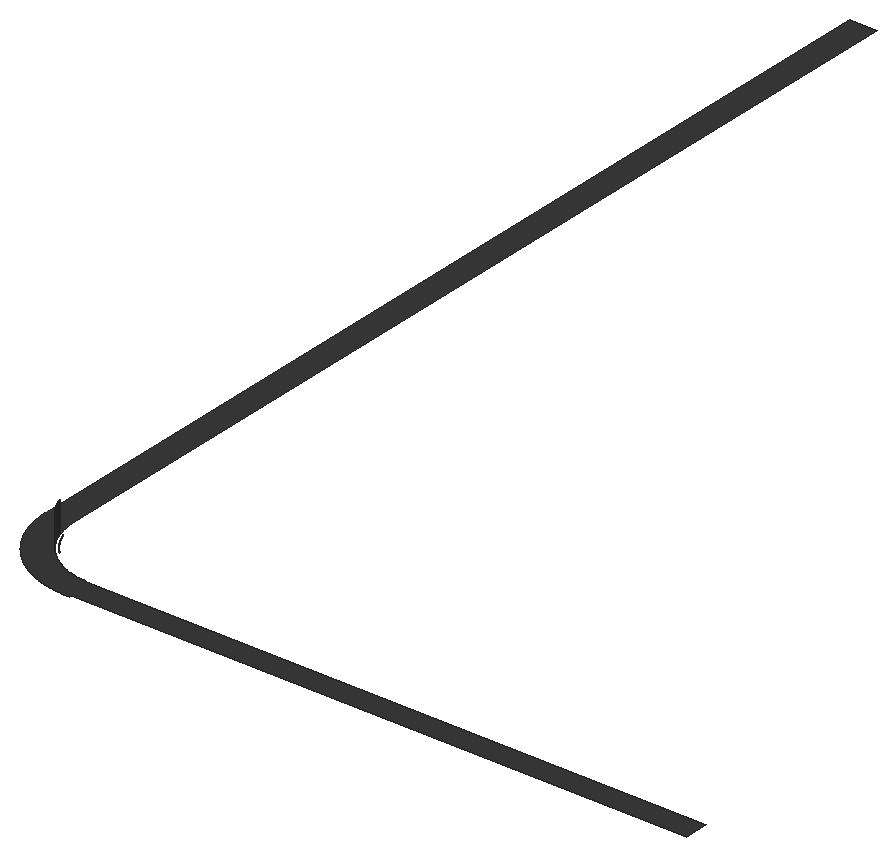
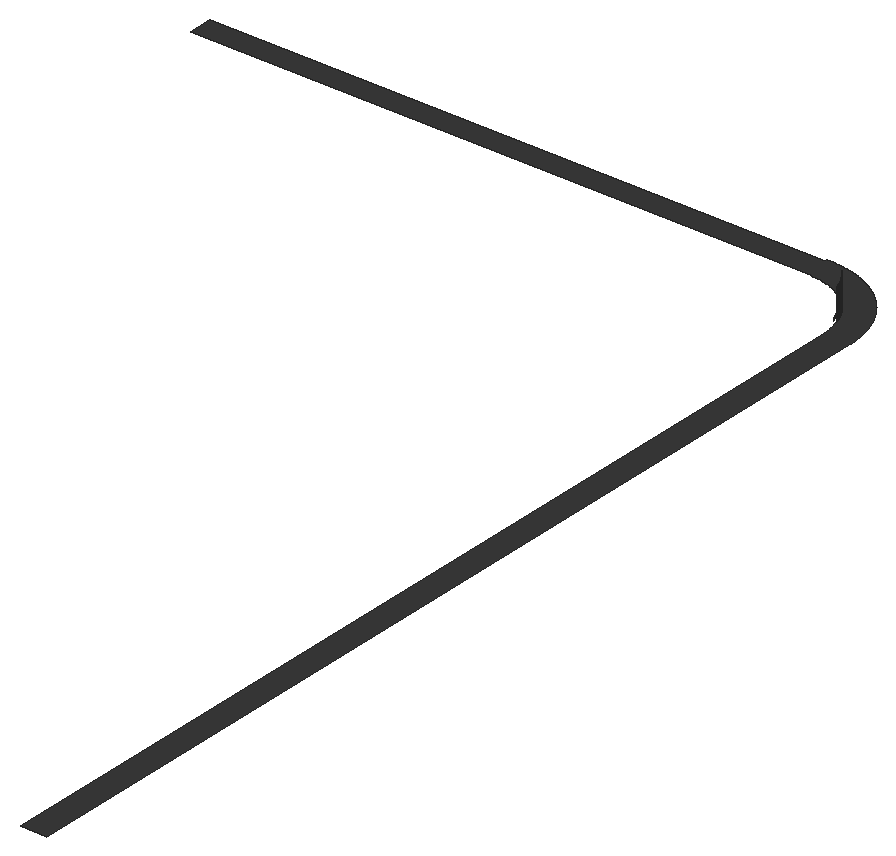
# SketchUp Ruby script. Lengths in inches.
U = 1.inch
M = Sketchup.active_model
def pt(a) = Geom::Point3d.new(a.map { |v| v * U })
def face(e, loops, mat)
  f = e.add_face(loops[0].map { |a| pt(a) })
  loops[1..].each { |l| e.add_face(l.map { |a| pt(a) }).erase! }
  f.material = f.back_material = mat if mat
  f
end
# faces: each face lists its corners as indices into pts; further lists are holes
def faces(e, pts, list, mat = nil) = list.each { |f| face(e, (f[0].is_a?(Array) ? f : [f]).map { |l| l.map { |i| pts[i] } }, mat) }
# xy, xz, yz: faces in a plane at the given z, y or x. An outline is a flat list of corners, or four numbers for a rectangle; further outlines are holes
def ring(l) = l.size == 4 ? [[l[0], l[1]], [l[2], l[1]], [l[2], l[3]], [l[0], l[3]]] : l.each_slice(2).to_a
def flat(e, list, mat, &to3) = list.each { |f| face(e, (f[0].is_a?(Array) ? f : [f]).map { |l| ring(l).map { |u, v| to3.(u, v) } }, mat) }
def xy(e, z, list, mat = nil) = flat(e, list, mat) { |x, y| [x, y, z] }
def xz(e, y, list, mat = nil) = flat(e, list, mat) { |x, z| [x, y, z] }
def yz(e, x, list, mat = nil) = flat(e, list, mat) { |y, z| [x, y, z] }
def lines(e, pts, list) = list.each { |a, b| e.add_line(pt(pts[a]), pt(pts[b])) }
# prism: a flat outline (further loops are holes) pulled along v
def prism(e, loops, v, mat = nil)
  f = face(e, loops, mat); d = Geom::Vector3d.new(v.map { |x| x * U })
  f.pushpull(f.normal.samedirection?(d) ? d.length : -d.length)
end
def box(e, o, s, mat = nil) = prism(e, [[o, [o[0] + s[0], o[1], o[2]], [o[0] + s[0], o[1] + s[1], o[2]], [o[0], o[1] + s[1], o[2]]]], [0, 0, s[2]], mat)
def at(x, y, z, deg = 0) = Geom::Transformation.translation(pt([x, y, z])) * Geom::Transformation.rotation(ORIGIN, Z_AXIS, deg.degrees)
def axes(o, x, y, z) = Geom::Transformation.new([*x, 0, *y, 0, *z, 0, *pt(o).to_a, 1])
def part(name) = M.definitions.add(name)
# library, detail: a bought-in or finely detailed component or shape, given as its bounding box
def library(name, o, s) = part(name).tap { |d| box(d.entities, o, s) }
def detail(e, o, s) = box(e.add_group.entities, o, s)
def put(e, d, t, mat = nil) = e.add_instance(d, t).tap { |i| i.material = mat if mat }
def group(e, t, mat = nil) = e.add_group.tap { |g| g.transformation = t; g.material = mat if mat }.entities
root = M.entities
M.materials.add("1496 AP 8293 CARBON COPY").color = [58, 58, 58]
xy(root,129,[[43.45,73,42.9,73.01,42.35,73.03,41.25,73.09,40.7,73.13,40.16,73.18,39.61,73.23,39.0625,73.29,38.52,73.36,37.97,73.43,36.35,73.7,35.27,73.92,34.73,74.04,34.2,74.16,33.66,74.29,33.13,74.43,32.07,74.73,31.55,74.89,31.02,75.06,30.5,75.23,29.98,75.41,29.46,75.6,28.95,75.79,28.4375,75.99,27.93,76.2,27.42,76.41,26.92,76.63,25.92,77.09,25.42,77.33,24.44,77.83,23.96,78.09,23.48,78.36,23,78.625,22.53,78.9,22.06,79.1875,21.59,79.48,21.125,79.78,20.67,80.08,20.21,80.39,19.76,80.7,19.3125,81.02,18.87,81.35,18.43,81.68,17.57,82.36,17.14,82.71,16.72,83.0625,16.31,83.42,15.49,84.16,15.09,84.53,14.69,84.92,14.3,85.3,13.92,85.69,13.53,86.09,13.16,86.49,12.42,87.31,12.0625,87.72,11.71,88.14,11.36,88.57,10.68,89.43,10.35,89.87,10.02,90.3125,9.7,90.76,9.39,91.21,9.08,91.67,8.78,92.125,8.48,92.59,8.1875,93.06,7.9,93.53,7.625,94,7.36,94.48,7.09,94.96,6.83,95.44,6.33,96.42,6.09,96.92,5.63,97.92,5.41,98.42,5.2,98.93,4.99,99.4375,4.79,99.95,4.6,100.46,4.41,100.98,4.23,101.5,4.06,102.02,3.89,102.55,3.73,103.07,3.43,104.13,3.29,104.66,3.16,105.2,3.04,105.73,2.92,106.27,2.7,107.35,2.43,108.97,2.36,109.52,2.29,110.0625,2.23,110.61,2.18,111.16,2.13,111.7,2.09,112.25,2.03,113.35,2.01,113.9,2,114.45,2,564,14,564,14,114.61,14.01,114.21,14.02,113.82,14.04,113.43,14.0625,113.04,14.09,112.65,14.125,112.25,14.16,111.86,14.26,111.08,14.31,110.7,14.43,109.92,14.5,109.53,14.58,109.15,14.66,108.76,14.74,108.38,14.92,107.62,15.02,107.24,15.125,106.86,15.24,106.48,15.35,106.1,15.59,105.36,15.85,104.62,15.99,104.25,16.14,103.88,16.28,103.52,16.4375,103.16,16.59,102.8,16.76,102.44,16.92,102.08,17.09,101.73,17.45,101.03,17.64,100.69,17.83,100.34,18.02,100,18.22,99.66,18.42,99.33,18.63,98.99,18.84,98.66,19.06,98.33,19.28,98.01,19.5,97.6875,19.73,97.37,19.96,97.05,20.44,96.43,20.6875,96.12,20.93,95.82,21.1875,95.52,21.44,95.22,21.71,94.93,21.97,94.64,22.24,94.35,22.51,94.07,23.07,93.51,23.35,93.24,23.64,92.97,23.93,92.71,24.22,92.44,24.52,92.1875,24.82,91.93,25.12,91.6875,25.43,91.44,26.05,90.96,26.37,90.73,26.6875,90.5,27.01,90.28,27.33,90.06,27.66,89.84,27.99,89.63,28.33,89.42,28.66,89.22,29,89.02,29.34,88.83,29.69,88.64,30.03,88.45,30.73,88.09,31.08,87.92,31.44,87.76,31.8,87.59,32.16,87.4375,32.52,87.28,32.88,87.14,33.25,86.99,33.62,86.85,34.36,86.59,35.1,86.35,35.48,86.24,35.86,86.125,36.24,86.02,36.62,85.92,37.38,85.74,37.76,85.66,38.15,85.58,38.53,85.5,38.92,85.43,39.7,85.31,40.08,85.26,40.86,85.16,41.25,85.125,41.65,85.09,42.04,85.0625,42.43,85.04,42.82,85.02,43.21,85.01,43.61,85,321,85,321,74,46,74,46,73]],"1496 AP 8293 CARBON COPY")
p = [[23.59,95.11,129],[23.85,94.85,129],[23.85,94.85,129.5],[23.59,95.11,129.5],[21.71,94.93,129],[21.44,95.22,129],
  [21.44,95.22,143],[21.71,94.93,143],[23.33,95.38,129],[23.33,95.38,129.5],[21.1875,95.52,129],[21.1875,95.52,143],
  [23.07,95.65,129],[23.07,95.65,129.5],[20.93,95.82,129],[20.93,95.82,143],[22.82,95.93,129],[22.82,95.93,129.5],
  [20.6875,96.12,129],[20.6875,96.12,143],[22.57,96.21,129],[22.57,96.21,129.5],[20.44,96.43,129],[20.44,96.43,143],
  [22.33,96.49,129],[22.33,96.49,129.5],[20.2,96.74,129],[20.2,96.74,143],[22.09,96.78,129],[22.09,96.78,129.5],
  [19.96,97.05,129],[19.96,97.05,143],[21.85,97.0625,129],[21.85,97.0625,129.5],[19.73,97.37,129],[19.73,97.37,143],
  [21.62,97.36,129],[21.62,97.36,129.5],[19.5,97.6875,129],[19.5,97.6875,143],[21.39,97.65,129],[21.39,97.65,129.5],
  [19.28,98.01,129],[19.28,98.01,143],[21.16,97.95,129],[21.16,97.95,129.5],[20.94,98.25,129],[20.94,98.25,129.5],
  [19.06,98.33,129],[19.06,98.33,143],[20.73,98.55,129],[20.73,98.55,129.5],[18.84,98.66,129],[18.84,98.66,143],
  [20.51,98.86,129],[20.51,98.86,129.5],[18.63,98.99,129],[18.63,98.99,143],[20.3,99.17,129],[20.3,99.17,129.5],
  [18.42,99.33,129],[18.42,99.33,143],[20.1,99.48,129],[20.1,99.48,129.5],[18.22,99.66,129],[18.22,99.66,143],
  [19.9,99.79,129],[19.9,99.79,129.5],[18.02,100,129],[18.02,100,143],[19.7,100.11,129],[19.7,100.11,129.5],
  [17.83,100.34,129],[17.83,100.34,143],[19.51,100.43,129],[19.51,100.43,129.5],[17.64,100.69,129],[17.64,100.69,143],
  [19.32,100.75,129],[19.32,100.75,129.5],[17.45,101.03,129],[17.45,101.03,143],[19.13,101.07,129],[19.13,101.07,129.5],
  [17.27,101.38,129],[17.27,101.38,143],[18.95,101.4,129],[18.95,101.4,129.5],[17.09,101.73,129],[17.09,101.73,143],
  [18.78,101.73,129],[18.78,101.73,129.5],[16.92,102.08,129],[16.92,102.08,143],[18.61,102.0625,129],[18.61,102.0625,129.5],
  [16.76,102.44,129],[16.76,102.44,143],[18.4375,102.39,129],[18.4375,102.39,129.5],[16.59,102.8,129],[16.59,102.8,143],
  [18.28,102.73,129],[18.28,102.73,129.5],[18.12,103.07,129],[18.12,103.07,129.5],[16.4375,103.16,129],[16.4375,103.16,143],
  [17.96,103.41,129],[17.96,103.41,129.5],[16.28,103.52,129],[16.28,103.52,143],[17.8125,103.75,129],[17.8125,103.75,129.5],
  [16.14,103.88,129],[16.14,103.88,143],[17.67,104.09,129],[17.67,104.09,129.5],[15.99,104.25,129],[15.99,104.25,143],
  [17.53,104.4375,129],[17.53,104.4375,129.5],[15.85,104.62,129],[15.85,104.62,143],[17.39,104.79,129],[17.39,104.79,129.5],
  [15.72,104.99,129],[15.72,104.99,143],[17.26,105.14,129],[17.26,105.14,129.5],[21.71,94.93,138],[21.44,95.22,138],
  [21.44,95.22,129.5],[21.71,94.93,129.5],[21.1875,95.52,138],[21.1875,95.52,129.5],[20.93,95.82,138],[20.93,95.82,129.5],
  [20.6875,96.12,138],[20.6875,96.12,129.5],[20.44,96.43,138],[20.44,96.43,129.5],[20.2,96.74,138],[20.2,96.74,129.5],
  [19.96,97.05,138],[19.96,97.05,129.5],[19.73,97.37,138],[19.73,97.37,129.5],[19.5,97.6875,138],[19.5,97.6875,129.5],
  [19.28,98.01,138],[19.28,98.01,129.5],[19.06,98.33,138],[19.06,98.33,129.5],[18.84,98.66,138],[18.84,98.66,129.5],
  [18.63,98.99,138],[18.63,98.99,129.5],[18.42,99.33,138],[18.42,99.33,129.5],[18.22,99.66,138],[18.22,99.66,129.5],
  [18.02,100,138],[18.02,100,129.5],[17.83,100.34,138],[17.83,100.34,129.5],[17.64,100.69,138],[17.64,100.69,129.5],
  [17.45,101.03,138],[17.45,101.03,129.5],[17.27,101.38,138],[17.27,101.38,129.5],[17.09,101.73,138],[17.09,101.73,129.5],
  [16.92,102.08,138],[16.92,102.08,129.5],[16.76,102.44,138],[16.76,102.44,129.5],[16.59,102.8,138],[16.59,102.8,129.5],
  [16.4375,103.16,138],[16.4375,103.16,129.5],[16.28,103.52,138],[16.28,103.52,129.5],[16.14,103.88,138],[16.14,103.88,129.5],
  [15.99,104.25,138],[15.99,104.25,129.5],[15.85,104.62,138],[15.85,104.62,129.5],[15.72,104.99,138],[15.72,104.99,129.5],
  [15.59,105.36,138],[15.59,105.36,129.5]]
faces(root,p,[[0,1,2,3],[8,0,3,9],[12,8,9,13],[16,12,13,17],[20,16,17,21],[24,20,21,25],[28,24,25,29],[32,28,29,33],
  [36,32,33,37],[40,36,37,41],[44,40,41,45],[46,44,45,47],[50,46,47,51],[54,50,51,55],[58,54,55,59],[62,58,59,63],
  [66,62,63,67],[70,66,67,71],[74,70,71,75],[78,74,75,79],[82,78,79,83],[86,82,83,87],[90,86,87,91],[94,90,91,95],
  [98,94,95,99],[102,98,99,103],[104,102,103,105],[108,104,105,109],[112,108,109,113],[116,112,113,117],[120,116,117,121],[124,120,121,125],
  [128,124,125,129],[130,131,132,133],[131,134,135,132],[134,136,137,135],[136,138,139,137],[138,140,141,139],[140,142,143,141],[142,144,145,143],
  [144,146,147,145],[146,148,149,147],[148,150,151,149],[150,152,153,151],[152,154,155,153],[154,156,157,155],[156,158,159,157],[158,160,161,159],
  [160,162,163,161],[162,164,165,163],[164,166,167,165],[166,168,169,167],[168,170,171,169],[170,172,173,171],[172,174,175,173],[174,176,177,175],
  [176,178,179,177],[178,180,181,179],[180,182,183,181],[182,184,185,183],[184,186,187,185],[186,188,189,187],[188,190,191,189],[190,192,193,191]])
faces(root,p,[[4,5,6,7],[5,10,11,6],[10,14,15,11],[14,18,19,15],[18,22,23,19],[22,26,27,23],[26,30,31,27],[30,34,35,31],
  [34,38,39,35],[38,42,43,39],[42,48,49,43],[48,52,53,49],[52,56,57,53],[56,60,61,57],[60,64,65,61],[64,68,69,65],
  [68,72,73,69],[72,76,77,73],[76,80,81,77],[80,84,85,81],[84,88,89,85],[88,92,93,89],[92,96,97,93],[96,100,101,97],
  [100,106,107,101],[106,110,111,107],[110,114,115,111],[114,118,119,115],[118,122,123,119],[122,126,127,123]],"1496 AP 8293 CARBON COPY")
